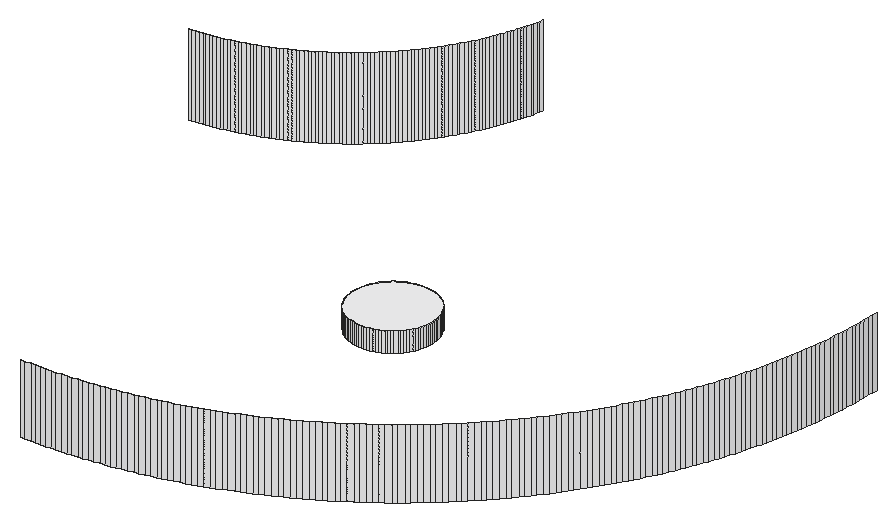
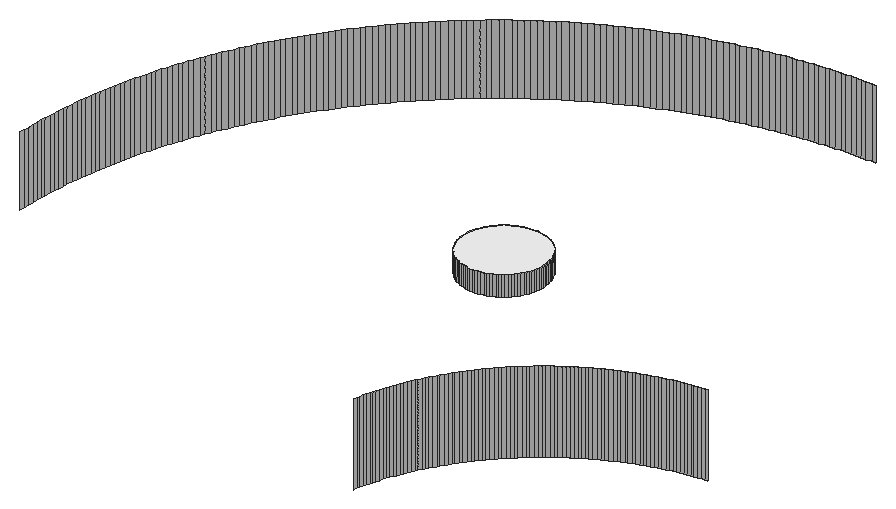
# SketchUp Ruby script. Lengths in inches.
U = 1.inch
M = Sketchup.active_model
def pt(a) = Geom::Point3d.new(a.map { |v| v * U })
def face(e, loops, mat)
  f = e.add_face(loops[0].map { |a| pt(a) })
  loops[1..].each { |l| e.add_face(l.map { |a| pt(a) }).erase! }
  f.material = f.back_material = mat if mat
  f
end
# faces: each face lists its corners as indices into pts; further lists are holes
def faces(e, pts, list, mat = nil) = list.each { |f| face(e, (f[0].is_a?(Array) ? f : [f]).map { |l| l.map { |i| pts[i] } }, mat) }
# xy, xz, yz: faces in a plane at the given z, y or x. An outline is a flat list of corners, or four numbers for a rectangle; further outlines are holes
def ring(l) = l.size == 4 ? [[l[0], l[1]], [l[2], l[1]], [l[2], l[3]], [l[0], l[3]]] : l.each_slice(2).to_a
def flat(e, list, mat, &to3) = list.each { |f| face(e, (f[0].is_a?(Array) ? f : [f]).map { |l| ring(l).map { |u, v| to3.(u, v) } }, mat) }
def xy(e, z, list, mat = nil) = flat(e, list, mat) { |x, y| [x, y, z] }
def xz(e, y, list, mat = nil) = flat(e, list, mat) { |x, z| [x, y, z] }
def yz(e, x, list, mat = nil) = flat(e, list, mat) { |y, z| [x, y, z] }
def lines(e, pts, list) = list.each { |a, b| e.add_line(pt(pts[a]), pt(pts[b])) }
# prism: a flat outline (further loops are holes) pulled along v
def prism(e, loops, v, mat = nil)
  f = face(e, loops, mat); d = Geom::Vector3d.new(v.map { |x| x * U })
  f.pushpull(f.normal.samedirection?(d) ? d.length : -d.length)
end
def box(e, o, s, mat = nil) = prism(e, [[o, [o[0] + s[0], o[1], o[2]], [o[0] + s[0], o[1] + s[1], o[2]], [o[0], o[1] + s[1], o[2]]]], [0, 0, s[2]], mat)
def at(x, y, z, deg = 0) = Geom::Transformation.translation(pt([x, y, z])) * Geom::Transformation.rotation(ORIGIN, Z_AXIS, deg.degrees)
def axes(o, x, y, z) = Geom::Transformation.new([*x, 0, *y, 0, *z, 0, *pt(o).to_a, 1])
def part(name) = M.definitions.add(name)
# library, detail: a bought-in or finely detailed component or shape, given as its bounding box
def library(name, o, s) = part(name).tap { |d| box(d.entities, o, s) }
def detail(e, o, s) = box(e.add_group.entities, o, s)
def put(e, d, t, mat = nil) = e.add_instance(d, t).tap { |i| i.material = mat if mat }
def group(e, t, mat = nil) = e.add_group.tap { |g| g.transformation = t; g.material = mat if mat }.entities
root = M.entities
M.materials.add("[Quartz Light Grey]").color = [251, 251, 252]
xy(root,112.81,[[182.9,56,182.77,56.01,182.65,56.03,182.52,56.06,182.4,56.09,182.28,56.13,182.17,56.18,181.95,56.3,181.84,56.37,181.74,56.45,181.65,56.53,181.47,56.71,181.39,56.81,181.32,56.91,181.2,57.13,181.15,57.24,181.1,57.36,181.04,57.6,181.02,57.73,181.01,57.85,181,57.98,181,58.1,181.01,58.23,181.03,58.35,181.06,58.48,181.09,58.6,181.13,58.72,181.18,58.83,181.3,59.05,181.37,59.16,181.45,59.26,181.53,59.35,181.71,59.53,181.81,59.61,181.91,59.68,182.13,59.8,182.24,59.85,182.36,59.9,182.6,59.96,182.73,59.98,182.85,59.99,182.98,60,183.1,60,183.23,59.99,183.35,59.97,183.48,59.94,183.6,59.91,183.72,59.87,183.83,59.82,184.05,59.7,184.16,59.63,184.26,59.55,184.35,59.47,184.53,59.29,184.61,59.19,184.68,59.09,184.8,58.87,184.85,58.76,184.9,58.64,184.96,58.4,184.98,58.27,184.99,58.15,185,58.02,185,57.9,184.99,57.77,184.97,57.65,184.94,57.52,184.91,57.4,184.87,57.28,184.82,57.17,184.7,56.95,184.63,56.84,184.55,56.74,184.47,56.65,184.29,56.47,184.19,56.39,184.09,56.32,183.87,56.2,183.76,56.15,183.64,56.1,183.4,56.04,183.27,56.02,183.15,56.01,183.02,56]],"[Quartz Light Grey]")
xz(root,42,[[177,111.81,177.25,115.32]],"[Quartz Light Grey]")
xz(root,42.01,[[177.5,111.81,177.75,115.32]],"[Quartz Light Grey]")
xz(root,56,[[182.9,111.81,183.02,112.81]],"[Quartz Light Grey]")
xz(root,60,[[182.98,111.81,183.1,112.81]],"[Quartz Light Grey]")
yz(root,181,[[57.98,111.81,58.1,112.81]],"[Quartz Light Grey]")
yz(root,185,[[57.9,111.81,58.02,112.81]],"[Quartz Light Grey]")
yz(root,200.99,[[65.25,111.81,65.5,115.32]],"[Quartz Light Grey]")
yz(root,201,[[65.75,111.81,66,115.32]],"[Quartz Light Grey]")
p = [[177.25,42,111.81],[177.5,42.01,111.81],[177.5,42.01,115.32],[177.25,42,115.32],[177.75,42.01,111.81],[178.01,42.02,111.81],
  [178.01,42.02,115.32],[177.75,42.01,115.32],[178.26,42.03,111.81],[178.26,42.03,115.32],[178.51,42.05,111.81],[178.51,42.05,115.32],
  [178.76,42.0625,111.81],[178.76,42.0625,115.32],[179.01,42.08,111.81],[179.01,42.08,115.32],[179.26,42.11,111.81],[179.26,42.11,115.32],
  [179.51,42.13,111.81],[179.51,42.13,115.32],[179.76,42.16,111.81],[179.76,42.16,115.32],[180.01,42.1875,111.81],[180.01,42.1875,115.32],
  [180.26,42.22,111.81],[180.26,42.22,115.32],[180.51,42.26,111.81],[180.51,42.26,115.32],[180.75,42.3,111.81],[180.75,42.3,115.32],
  [181,42.34,111.81],[181,42.34,115.32],[181.25,42.38,111.81],[181.25,42.38,115.32],[181.5,42.43,111.81],[181.5,42.43,115.32],
  [181.74,42.47,111.81],[181.74,42.47,115.32],[181.99,42.52,111.81],[181.99,42.52,115.32],[182.24,42.58,111.81],[182.24,42.58,115.32],
  [182.48,42.63,111.81],[182.48,42.63,115.32],[182.72,42.69,111.81],[182.72,42.69,115.32],[182.97,42.75,111.81],[182.97,42.75,115.32],
  [183.21,42.82,111.81],[183.21,42.82,115.32],[183.45,42.88,111.81],[183.45,42.88,115.32],[183.7,42.95,111.81],[183.7,42.95,115.32],
  [183.9375,43.02,111.81],[183.9375,43.02,115.32],[184.18,43.1,111.81],[184.18,43.1,115.32],[184.42,43.17,111.81],[184.42,43.17,115.32],
  [184.66,43.25,111.81],[184.66,43.25,115.32],[184.89,43.33,111.81],[184.89,43.33,115.32],[185.13,43.42,111.81],[185.13,43.42,115.32],
  [185.37,43.51,111.81],[185.37,43.51,115.32],[185.6,43.59,111.81],[185.6,43.59,115.32],[185.83,43.69,111.81],[185.83,43.69,115.32],
  [186.07,43.78,111.81],[186.07,43.78,115.32],[186.3,43.875,111.81],[186.3,43.875,115.32],[186.53,43.97,111.81],[186.53,43.97,115.32],
  [186.76,44.07,111.81],[186.76,44.07,115.32],[186.99,44.18,111.81],[186.99,44.18,115.32],[187.22,44.28,111.81],[187.22,44.28,115.32],
  [187.45,44.39,111.81],[187.45,44.39,115.32],[187.67,44.5,111.81],[187.67,44.5,115.32],[187.9,44.62,111.81],[187.9,44.62,115.32],
  [188.12,44.73,111.81],[188.12,44.73,115.32],[188.34,44.85,111.81],[188.34,44.85,115.32],[188.5625,44.97,111.81],[188.5625,44.97,115.32],
  [188.78,45.09,111.81],[188.78,45.09,115.32],[189,45.22,111.81],[189,45.22,115.32],[189.22,45.34,111.81],[189.22,45.34,115.32],
  [189.43,45.47,111.81],[189.43,45.47,115.32],[189.65,45.6,111.81],[189.65,45.6,115.32],[189.86,45.74,111.81],[189.86,45.74,115.32],
  [190.07,45.87,111.81],[190.07,45.87,115.32],[190.28,46.01,111.81],[190.28,46.01,115.32],[190.49,46.15,111.81],[190.49,46.15,115.32],
  [190.7,46.29,111.81],[190.7,46.29,115.32],[190.9,46.4375,111.81],[190.9,46.4375,115.32],[191.11,46.58,111.81],[191.11,46.58,115.32],
  [191.31,46.73,111.81],[191.31,46.73,115.32],[191.51,46.88,111.81],[191.51,46.88,115.32],[191.71,47.04,111.81],[191.71,47.04,115.32],
  [191.91,47.19,111.81],[191.91,47.19,115.32],[192.1,47.35,111.81],[192.1,47.35,115.32],[192.3,47.51,111.81],[192.3,47.51,115.32],
  [192.49,47.67,111.81],[192.49,47.67,115.32],[192.68,47.83,111.81],[192.68,47.83,115.32],[192.87,48,111.81],[192.87,48,115.32],
  [193.06,48.16,111.81],[193.06,48.16,115.32],[193.25,48.33,111.81],[193.25,48.33,115.32],[193.43,48.5,111.81],[193.43,48.5,115.32],
  [193.61,48.68,111.81],[193.61,48.68,115.32],[193.79,48.85,111.81],[193.79,48.85,115.32],[193.97,49.03,111.81],[193.97,49.03,115.32],
  [194.15,49.21,111.81],[194.15,49.21,115.32],[194.32,49.39,111.81],[194.32,49.39,115.32],[194.5,49.57,111.81],[194.5,49.57,115.32],
  [194.67,49.75,111.81],[194.67,49.75,115.32],[194.84,49.94,111.81],[194.84,49.94,115.32],[195,50.13,111.81],[195,50.13,115.32],
  [195.17,50.32,111.81],[195.17,50.32,115.32],[195.33,50.51,111.81],[195.33,50.51,115.32],[195.49,50.7,111.81],[195.49,50.7,115.32],
  [195.65,50.9,111.81],[195.65,50.9,115.32],[195.81,51.09,111.81],[195.81,51.09,115.32],[195.96,51.29,111.81],[195.96,51.29,115.32],
  [196.12,51.49,111.81],[196.12,51.49,115.32],[196.27,51.69,111.81],[196.27,51.69,115.32],[196.42,51.89,111.81],[196.42,51.89,115.32],
  [196.5625,52.1,111.81],[196.5625,52.1,115.32],[196.71,52.3,111.81],[196.71,52.3,115.32],[196.85,52.51,111.81],[196.85,52.51,115.32],
  [196.99,52.72,111.81],[196.99,52.72,115.32],[197.13,52.93,111.81],[197.13,52.93,115.32],[197.26,53.14,111.81],[197.26,53.14,115.32],
  [197.4,53.35,111.81],[197.4,53.35,115.32],[197.53,53.57,111.81],[197.53,53.57,115.32],[197.66,53.78,111.81],[197.66,53.78,115.32],
  [197.78,54,111.81],[197.78,54,115.32],[197.91,54.22,111.81],[197.91,54.22,115.32],[198.03,54.4375,111.81],[198.03,54.4375,115.32],
  [198.15,54.66,111.81],[198.15,54.66,115.32],[198.27,54.88,111.81],[198.27,54.88,115.32],[198.38,55.1,111.81],[198.38,55.1,115.32],
  [198.5,55.33,111.81],[198.5,55.33,115.32],[198.61,55.55,111.81],[198.61,55.55,115.32],[198.72,55.78,111.81],[198.72,55.78,115.32],
  [198.82,56.01,111.81],[198.82,56.01,115.32],[182.65,56.03,111.81],[182.52,56.06,111.81],[182.52,56.06,112.81],[182.65,56.03,112.81],
  [182.77,56.01,111.81],[182.77,56.01,112.81],[182.9,56,111.81],[182.9,56,112.81],[183.15,56.01,111.81],[183.02,56,111.81],
  [183.02,56,112.81],[183.15,56.01,112.81],[183.27,56.02,111.81],[183.27,56.02,112.81],[183.4,56.04,111.81],[183.4,56.04,112.81],
  [183.52,56.07,111.81],[183.52,56.07,112.81],[198.93,56.24,111.81],[198.93,56.24,115.32],[182.28,56.13,111.81],[182.17,56.18,111.81],
  [182.17,56.18,112.81],[182.28,56.13,112.81],[182.4,56.09,111.81],[182.4,56.09,112.81],[183.64,56.1,111.81],[183.64,56.1,112.81],
  [183.76,56.15,111.81],[183.76,56.15,112.81],[183.87,56.2,111.81],[183.87,56.2,112.81],[182.06,56.24,111.81],[181.95,56.3,111.81],
  [181.95,56.3,112.81],[182.06,56.24,112.81],[183.98,56.26,111.81],[183.98,56.26,112.81],[199.03,56.47,111.81],[199.03,56.47,115.32],
  [181.84,56.37,111.81],[181.84,56.37,112.81],[184.09,56.32,111.81],[184.09,56.32,112.81],[184.19,56.39,111.81],[184.19,56.39,112.81],
  [181.74,56.45,111.81],[181.65,56.53,111.81],[181.65,56.53,112.81],[181.74,56.45,112.81],[184.29,56.47,111.81],[184.29,56.47,112.81],
  [181.56,56.62,111.81],[181.56,56.62,112.81],[184.38,56.56,111.81],[184.38,56.56,112.81],[199.125,56.7,111.81],[199.125,56.7,115.32],
  [181.47,56.71,111.81],[181.47,56.71,112.81],[184.47,56.65,111.81],[184.47,56.65,112.81],[184.55,56.74,111.81],[184.55,56.74,112.81],
  [181.39,56.81,111.81],[181.39,56.81,112.81],[184.63,56.84,111.81],[184.63,56.84,112.81],[199.22,56.93,111.81],[199.22,56.93,115.32],
  [181.32,56.91,111.81],[181.32,56.91,112.81],[184.7,56.95,111.81],[184.7,56.95,112.81],[181.26,57.02,111.81],[181.26,57.02,112.81],
  [184.76,57.06,111.81],[184.76,57.06,112.81],[199.31,57.17,111.81],[199.31,57.17,115.32],[181.2,57.13,111.81],[181.2,57.13,112.81],
  [181.15,57.24,111.81],[181.15,57.24,112.81],[184.82,57.17,111.81],[184.82,57.17,112.81],[181.1,57.36,111.81],[181.1,57.36,112.81],
  [184.87,57.28,111.81],[184.87,57.28,112.81],[199.41,57.4,111.81],[199.41,57.4,115.32],[184.91,57.4,111.81],[184.91,57.4,112.81],
  [181.07,57.48,111.81],[181.07,57.48,112.81],[184.94,57.52,111.81],[184.94,57.52,112.81],[199.49,57.63,111.81],[199.49,57.63,115.32],
  [181.04,57.6,111.81],[181.04,57.6,112.81],[184.97,57.65,111.81],[184.97,57.65,112.81],[181.02,57.73,111.81],[181.02,57.73,112.81],
  [184.99,57.77,111.81],[184.99,57.77,112.81],[199.58,57.87,111.81],[199.58,57.87,115.32],[181.01,57.85,111.81],[181.01,57.85,112.81],
  [185,57.9,111.81],[185,57.9,112.81],[181,57.98,111.81],[181,57.98,112.81],[199.67,58.11,111.81],[199.67,58.11,115.32],
  [184.99,58.15,111.81],[185,58.02,111.81],[185,58.02,112.81],[184.99,58.15,112.81],[181,58.1,111.81],[181.01,58.23,111.81],
  [181.01,58.23,112.81],[181,58.1,112.81],[184.98,58.27,111.81],[184.98,58.27,112.81],[199.75,58.34,111.81],[199.75,58.34,115.32],
  [181.03,58.35,111.81],[181.03,58.35,112.81],[184.96,58.4,111.81],[184.96,58.4,112.81],[199.83,58.58,111.81],[199.83,58.58,115.32],
  [181.06,58.48,111.81],[181.06,58.48,112.81],[184.93,58.52,111.81],[184.93,58.52,112.81],[181.09,58.6,111.81],[181.09,58.6,112.81],
  [184.9,58.64,111.81],[184.9,58.64,112.81],[181.13,58.72,111.81],[181.13,58.72,112.81],[184.85,58.76,111.81],[184.85,58.76,112.81],
  [199.9,58.82,111.81],[199.9,58.82,115.32],[181.18,58.83,111.81],[181.18,58.83,112.81],[181.24,58.94,111.81],[181.24,58.94,112.81],
  [184.8,58.87,111.81],[184.8,58.87,112.81],[199.98,59.0625,111.81],[199.98,59.0625,115.32],[181.3,59.05,111.81],[181.3,59.05,112.81],
  [184.74,58.98,111.81],[184.74,58.98,112.81],[184.68,59.09,111.81],[184.68,59.09,112.81],[181.37,59.16,111.81],[181.37,59.16,112.81],
  [184.61,59.19,111.81],[184.61,59.19,112.81],[200.05,59.3,111.81],[200.05,59.3,115.32],[181.45,59.26,111.81],[181.45,59.26,112.81],
  [184.53,59.29,111.81],[184.53,59.29,112.81],[181.53,59.35,111.81],[181.53,59.35,112.81],[184.44,59.38,111.81],[184.44,59.38,112.81],
  [200.12,59.55,111.81],[200.12,59.55,115.32],[181.62,59.44,111.81],[181.62,59.44,112.81],[181.71,59.53,111.81],[181.71,59.53,112.81],
  [184.35,59.47,111.81],[184.35,59.47,112.81],[181.81,59.61,111.81],[181.81,59.61,112.81],[184.26,59.55,111.81],[184.26,59.55,112.81],
  [200.18,59.79,111.81],[200.18,59.79,115.32],[181.91,59.68,111.81],[181.91,59.68,112.81],[184.05,59.7,111.81],[184.16,59.63,111.81],
  [184.16,59.63,112.81],[184.05,59.7,112.81],[182.02,59.74,111.81],[182.02,59.74,112.81],[182.13,59.8,111.81],[182.13,59.8,112.81],
  [183.94,59.76,111.81],[183.94,59.76,112.81],[182.24,59.85,111.81],[182.24,59.85,112.81],[183.72,59.87,111.81],[183.83,59.82,111.81],
  [183.83,59.82,112.81],[183.72,59.87,112.81],[200.25,60.03,111.81],[200.25,60.03,115.32],[182.36,59.9,111.81],[182.36,59.9,112.81],
  [182.48,59.93,111.81],[182.48,59.93,112.81],[182.6,59.96,111.81],[182.6,59.96,112.81],[183.35,59.97,111.81],[183.48,59.94,111.81],
  [183.48,59.94,112.81],[183.35,59.97,112.81],[183.6,59.91,111.81],[183.6,59.91,112.81],[182.73,59.98,111.81],[182.73,59.98,112.81],
  [182.85,59.99,111.81],[182.85,59.99,112.81],[182.98,60,111.81],[182.98,60,112.81],[183.1,60,111.81],[183.23,59.99,111.81],
  [183.23,59.99,112.81],[183.1,60,112.81],[200.31,60.28,111.81],[200.31,60.28,115.32],[200.37,60.52,111.81],[200.37,60.52,115.32],
  [200.42,60.76,111.81],[200.42,60.76,115.32],[200.48,61.01,111.81],[200.48,61.01,115.32],[200.53,61.26,111.81],[200.53,61.26,115.32],
  [200.57,61.5,111.81],[200.57,61.5,115.32],[200.62,61.75,111.81],[200.62,61.75,115.32],[200.66,62,111.81],[200.66,62,115.32],
  [200.7,62.25,111.81],[200.7,62.25,115.32],[200.74,62.49,111.81],[200.74,62.49,115.32],[200.78,62.74,111.81],[200.78,62.74,115.32],
  [200.8125,62.99,111.81],[200.8125,62.99,115.32],[200.84,63.24,111.81],[200.84,63.24,115.32],[200.87,63.49,111.81],[200.87,63.49,115.32],
  [200.89,63.74,111.81],[200.89,63.74,115.32],[200.92,63.99,111.81],[200.92,63.99,115.32],[200.9375,64.24,111.81],[200.9375,64.24,115.32],
  [200.95,64.49,111.81],[200.95,64.49,115.32],[200.97,64.74,111.81],[200.97,64.74,115.32],[200.98,64.99,111.81],[200.98,64.99,115.32],
  [200.99,65.25,111.81],[200.99,65.25,115.32],[200.99,65.5,111.81],[201,65.75,111.81],[201,65.75,115.32],[200.99,65.5,115.32],
  [166.41,66.08,111.81],[166.25,66.07,111.81],[166.25,66.07,115.91],[166.41,66.08,115.91],[166.57,66.1,111.81],[166.57,66.1,115.91],
  [166.72,66.125,111.81],[166.72,66.125,115.91],[166.88,66.15,111.81],[166.88,66.15,115.91],[167.03,66.17,111.81],[167.03,66.17,115.91],
  [167.1875,66.2,111.81],[167.1875,66.2,115.91],[167.34,66.23,111.81],[167.34,66.23,115.91],[167.49,66.26,111.81],[167.49,66.26,115.91],
  [167.65,66.3,111.81],[167.65,66.3,115.91],[167.8,66.33,111.81],[167.8,66.33,115.91],[167.95,66.37,111.81],[167.95,66.37,115.91],
  [168.11,66.41,111.81],[168.11,66.41,115.91],[168.26,66.45,111.81],[168.26,66.45,115.91],[168.41,66.49,111.81],[168.41,66.49,115.91],
  [168.56,66.54,111.81],[168.56,66.54,115.91],[168.71,66.59,111.81],[168.71,66.59,115.91],[168.86,66.64,111.81],[168.86,66.64,115.91],
  [169.01,66.6875,111.81],[169.01,66.6875,115.91],[169.15,66.74,111.81],[169.15,66.74,115.91],[169.3,66.8,111.81],[169.3,66.8,115.91],
  [169.45,66.85,111.81],[169.45,66.85,115.91],[169.59,66.91,111.81],[169.59,66.91,115.91],[169.74,66.97,111.81],[169.74,66.97,115.91],
  [169.88,67.04,111.81],[169.88,67.04,115.91],[170.02,67.1,111.81],[170.02,67.1,115.91],[170.17,67.17,111.81],[170.17,67.17,115.91],
  [170.31,67.24,111.81],[170.31,67.24,115.91],[170.45,67.31,111.81],[170.45,67.31,115.91],[170.59,67.38,111.81],[170.59,67.38,115.91],
  [170.73,67.45,111.81],[170.73,67.45,115.91],[170.86,67.53,111.81],[170.86,67.53,115.91],[171,67.61,111.81],[171,67.61,115.91],
  [171.14,67.6875,111.81],[171.14,67.6875,115.91],[171.27,67.77,111.81],[171.27,67.77,115.91],[171.4,67.85,111.81],[171.4,67.85,115.91],
  [171.54,67.9375,111.81],[171.54,67.9375,115.91],[171.67,68.02,111.81],[171.67,68.02,115.91],[171.8,68.11,111.81],[171.8,68.11,115.91],
  [171.93,68.2,111.81],[171.93,68.2,115.91],[172.05,68.29,111.81],[172.05,68.29,115.91],[172.18,68.38,111.81],[172.18,68.38,115.91],
  [172.31,68.48,111.81],[172.31,68.48,115.91],[172.43,68.58,111.81],[172.43,68.58,115.91],[172.55,68.67,111.81],[172.55,68.67,115.91],
  [172.67,68.77,111.81],[172.67,68.77,115.91],[172.79,68.875,111.81],[172.79,68.875,115.91],[172.91,68.98,111.81],[172.91,68.98,115.91],
  [173.03,69.08,111.81],[173.03,69.08,115.91],[173.15,69.1875,111.81],[173.15,69.1875,115.91],[173.26,69.3,111.81],[173.26,69.3,115.91],
  [173.375,69.4,111.81],[173.375,69.4,115.91],[173.49,69.51,111.81],[173.49,69.51,115.91],[173.6,69.625,111.81],[173.6,69.625,115.91],
  [173.7,69.74,111.81],[173.7,69.74,115.91],[173.8125,69.85,111.81],[173.8125,69.85,115.91],[173.92,69.97,111.81],[173.92,69.97,115.91],
  [174.02,70.09,111.81],[174.02,70.09,115.91],[174.125,70.21,111.81],[174.125,70.21,115.91],[174.23,70.33,111.81],[174.23,70.33,115.91],
  [174.33,70.45,111.81],[174.33,70.45,115.91],[174.42,70.57,111.81],[174.42,70.57,115.91],[174.52,70.69,111.81],[174.52,70.69,115.91],
  [174.62,70.82,111.81],[174.62,70.82,115.91],[174.71,70.95,111.81],[174.71,70.95,115.91],[174.8,71.07,111.81],[174.8,71.07,115.91],
  [174.89,71.2,111.81],[174.89,71.2,115.91],[174.98,71.33,111.81],[174.98,71.33,115.91],[175.0625,71.46,111.81],[175.0625,71.46,115.91],
  [175.15,71.6,111.81],[175.15,71.6,115.91],[175.23,71.73,111.81],[175.23,71.73,115.91],[175.3125,71.86,111.81],[175.3125,71.86,115.91],
  [175.39,72,111.81],[175.39,72,115.91],[175.47,72.14,111.81],[175.47,72.14,115.91],[175.55,72.27,111.81],[175.55,72.27,115.91],
  [175.62,72.41,111.81],[175.62,72.41,115.91],[175.69,72.55,111.81],[175.69,72.55,115.91],[175.76,72.69,111.81],[175.76,72.69,115.91],
  [175.83,72.83,111.81],[175.83,72.83,115.91],[175.9,72.98,111.81],[175.9,72.98,115.91],[175.96,73.12,111.81],[175.96,73.12,115.91],
  [176.03,73.26,111.81],[176.03,73.26,115.91],[176.09,73.41,111.81],[176.09,73.41,115.91],[176.15,73.55,111.81],[176.15,73.55,115.91],
  [176.2,73.7,111.81],[176.2,73.7,115.91],[176.26,73.85,111.81],[176.26,73.85,115.91],[176.3125,73.99,111.81],[176.3125,73.99,115.91],
  [176.36,74.14,111.81],[176.36,74.14,115.91],[176.41,74.29,111.81],[176.41,74.29,115.91],[176.46,74.44,111.81],[176.46,74.44,115.91],
  [176.51,74.59,111.81],[176.51,74.59,115.91],[176.55,74.74,111.81],[176.55,74.74,115.91],[176.59,74.89,111.81],[176.59,74.89,115.91],
  [176.63,75.05,111.81],[176.63,75.05,115.91],[176.67,75.2,111.81],[176.67,75.2,115.91],[176.7,75.35,111.81],[176.7,75.35,115.91]]
faces(root,p,[[0,1,2,3],[4,5,6,7],[5,8,9,6],[8,10,11,9],[10,12,13,11],[12,14,15,13],[14,16,17,15],[16,18,19,17],
  [18,20,21,19],[20,22,23,21],[22,24,25,23],[24,26,27,25],[26,28,29,27],[28,30,31,29],[30,32,33,31],[32,34,35,33],
  [34,36,37,35],[36,38,39,37],[38,40,41,39],[40,42,43,41],[42,44,45,43],[44,46,47,45],[46,48,49,47],[48,50,51,49],
  [50,52,53,51],[52,54,55,53],[54,56,57,55],[56,58,59,57],[58,60,61,59],[60,62,63,61],[62,64,65,63],[64,66,67,65],
  [66,68,69,67],[68,70,71,69],[70,72,73,71],[72,74,75,73],[74,76,77,75],[76,78,79,77],[78,80,81,79],[80,82,83,81],
  [82,84,85,83],[84,86,87,85],[86,88,89,87],[88,90,91,89],[90,92,93,91],[92,94,95,93],[94,96,97,95],[96,98,99,97],
  [98,100,101,99],[100,102,103,101],[102,104,105,103],[104,106,107,105],[106,108,109,107],[108,110,111,109],[110,112,113,111],[112,114,115,113],
  [114,116,117,115],[116,118,119,117],[118,120,121,119],[120,122,123,121],[122,124,125,123],[124,126,127,125],[126,128,129,127],[128,130,131,129],
  [130,132,133,131],[132,134,135,133],[134,136,137,135],[136,138,139,137],[138,140,141,139],[140,142,143,141],[142,144,145,143],[144,146,147,145],
  [146,148,149,147],[148,150,151,149],[150,152,153,151],[152,154,155,153],[154,156,157,155],[156,158,159,157],[158,160,161,159],[160,162,163,161],
  [162,164,165,163],[164,166,167,165],[166,168,169,167],[168,170,171,169],[170,172,173,171],[172,174,175,173],[174,176,177,175],[176,178,179,177],
  [178,180,181,179],[180,182,183,181],[182,184,185,183],[184,186,187,185],[186,188,189,187],[188,190,191,189],[190,192,193,191],[192,194,195,193],
  [194,196,197,195],[196,198,199,197],[198,200,201,199],[200,202,203,201],[202,204,205,203],[204,206,207,205],[206,208,209,207],[208,210,211,209],
  [210,212,213,211],[212,214,215,213],[214,216,217,215],[218,219,220,221],[222,218,221,223],[224,222,223,225],[226,227,228,229],[230,226,229,231],
  [232,230,231,233],[234,232,233,235],[216,236,237,217],[238,239,240,241],[242,238,241,243],[219,242,243,220],[244,234,235,245],[246,244,245,247],
  [248,246,247,249],[250,251,252,253],[239,250,253,240],[254,248,249,255],[236,256,257,237],[251,258,259,252],[260,254,255,261],[262,260,261,263],
  [264,265,266,267],[258,264,267,259],[268,262,263,269],[265,270,271,266],[272,268,269,273],[256,274,275,257],[270,276,277,271],[278,272,273,279],
  [280,278,279,281],[276,282,283,277],[284,280,281,285],[274,286,287,275],[282,288,289,283],[290,284,285,291],[288,292,293,289],[294,290,291,295],
  [286,296,297,287],[292,298,299,293],[298,300,301,299],[302,294,295,303],[300,304,305,301],[306,302,303,307],[296,308,309,297],[310,306,307,311],
  [304,312,313,305],[314,310,311,315],[308,316,317,309],[312,318,319,313],[320,314,315,321],[318,322,323,319],[324,320,321,325],[316,326,327,317],
  [322,328,329,323],[330,324,325,331],[328,332,333,329],[326,334,335,327],[336,337,338,339],[340,341,342,343],[344,336,339,345],[334,346,347,335],
  [341,348,349,342],[350,344,345,351],[346,352,353,347],[348,354,355,349],[356,350,351,357],[354,358,359,355],[360,356,357,361],[358,362,363,359],
  [364,360,361,365],[352,366,367,353],[362,368,369,363],[368,370,371,369],[372,364,365,373],[366,374,375,367],[370,376,377,371],[378,372,373,379],
  [380,378,379,381],[376,382,383,377],[384,380,381,385],[374,386,387,375],[382,388,389,383],[390,384,385,391],[388,392,393,389],[394,390,391,395],
  [386,396,397,387],[392,398,399,393],[398,400,401,399],[402,394,395,403],[400,404,405,401],[406,402,403,407],[396,408,409,397],[404,410,411,405],
  [412,413,414,415],[413,406,407,414],[410,416,417,411],[416,418,419,417],[420,412,415,421],[418,422,423,419],[424,425,426,427],[425,420,421,426],
  [408,428,429,409],[422,430,431,423],[430,432,433,431],[432,434,435,433],[436,437,438,439],[437,440,441,438],[440,424,427,441],[434,442,443,435],
  [442,444,445,443],[444,446,447,445],[448,449,450,451],[449,436,439,450],[428,452,453,429],[452,454,455,453],[454,456,457,455],[456,458,459,457],
  [458,460,461,459],[460,462,463,461],[462,464,465,463],[464,466,467,465],[466,468,469,467],[468,470,471,469],[470,472,473,471],[472,474,475,473],
  [474,476,477,475],[476,478,479,477],[478,480,481,479],[480,482,483,481],[482,484,485,483],[484,486,487,485],[486,488,489,487],[488,490,491,489],
  [490,492,493,491],[494,495,496,497],[498,499,500,501],[502,498,501,503],[504,502,503,505],[506,504,505,507],[508,506,507,509],[510,508,509,511],
  [512,510,511,513],[514,512,513,515],[516,514,515,517],[518,516,517,519],[520,518,519,521],[522,520,521,523],[524,522,523,525],[526,524,525,527],
  [528,526,527,529],[530,528,529,531],[532,530,531,533],[534,532,533,535],[536,534,535,537],[538,536,537,539],[540,538,539,541],[542,540,541,543],
  [544,542,543,545],[546,544,545,547],[548,546,547,549],[550,548,549,551],[552,550,551,553],[554,552,553,555],[556,554,555,557],[558,556,557,559],
  [560,558,559,561],[562,560,561,563],[564,562,563,565],[566,564,565,567],[568,566,567,569],[570,568,569,571],[572,570,571,573],[574,572,573,575],
  [576,574,575,577],[578,576,577,579],[580,578,579,581],[582,580,581,583],[584,582,583,585],[586,584,585,587],[588,586,587,589],[590,588,589,591],
  [592,590,591,593],[594,592,593,595],[596,594,595,597],[598,596,597,599],[600,598,599,601],[602,600,601,603],[604,602,603,605],[606,604,605,607],
  [608,606,607,609],[610,608,609,611],[612,610,611,613],[614,612,613,615],[616,614,615,617],[618,616,617,619],[620,618,619,621],[622,620,621,623],
  [624,622,623,625],[626,624,625,627],[628,626,627,629],[630,628,629,631],[632,630,631,633],[634,632,633,635],[636,634,635,637],[638,636,637,639],
  [640,638,639,641],[642,640,641,643],[644,642,643,645],[646,644,645,647],[648,646,647,649],[650,648,649,651],[652,650,651,653],[654,652,653,655],
  [656,654,655,657],[658,656,657,659],[660,658,659,661],[662,660,661,663],[664,662,663,665],[666,664,665,667],[668,666,667,669],[670,668,669,671],
  [672,670,671,673],[674,672,673,675],[676,674,675,677],[678,676,677,679],[680,678,679,681],[682,680,681,683],[684,682,683,685],[686,684,685,687],
  [688,686,687,689]],"[Quartz Light Grey]")
